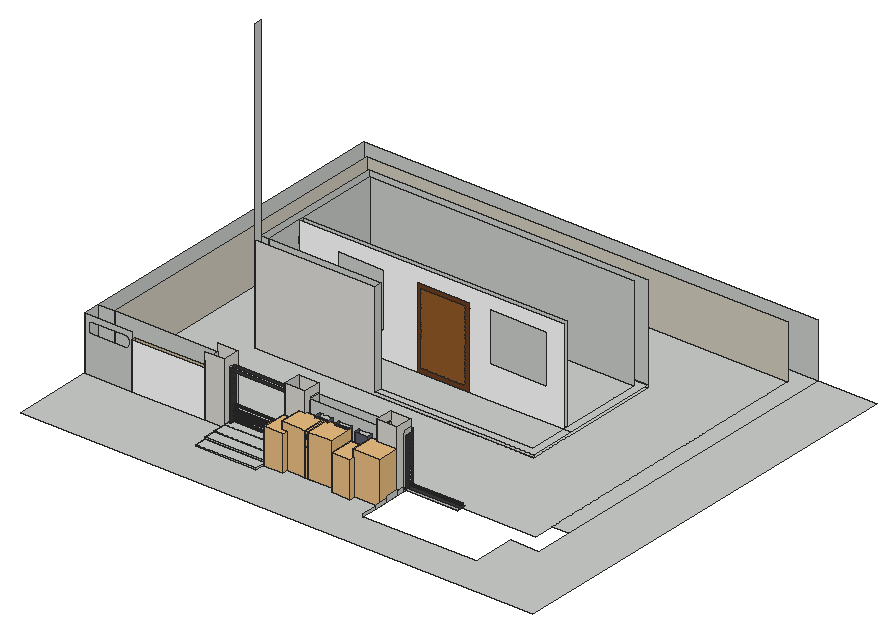
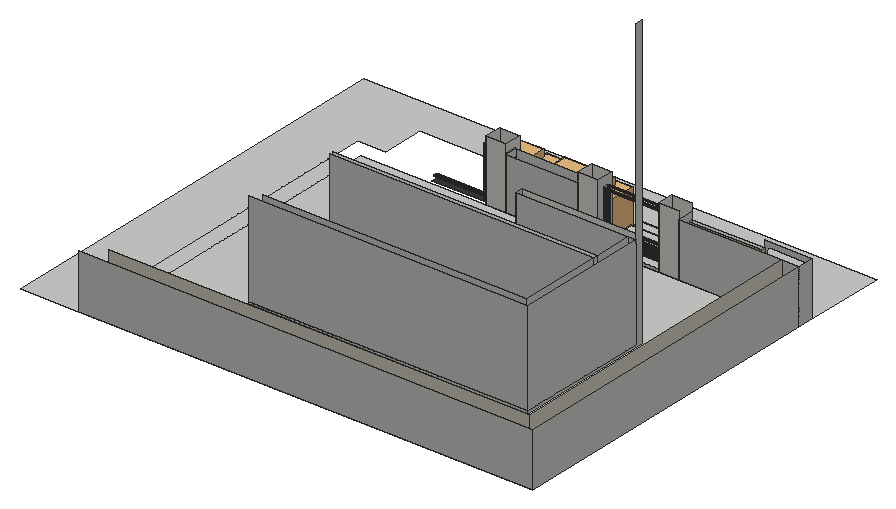
# SketchUp Ruby script. Lengths in inches.
U = 1.inch
M = Sketchup.active_model
def pt(a) = Geom::Point3d.new(a.map { |v| v * U })
def face(e, loops, mat)
  f = e.add_face(loops[0].map { |a| pt(a) })
  loops[1..].each { |l| e.add_face(l.map { |a| pt(a) }).erase! }
  f.material = f.back_material = mat if mat
  f
end
# faces: each face lists its corners as indices into pts; further lists are holes
def faces(e, pts, list, mat = nil) = list.each { |f| face(e, (f[0].is_a?(Array) ? f : [f]).map { |l| l.map { |i| pts[i] } }, mat) }
# xy, xz, yz: faces in a plane at the given z, y or x. An outline is a flat list of corners, or four numbers for a rectangle; further outlines are holes
def ring(l) = l.size == 4 ? [[l[0], l[1]], [l[2], l[1]], [l[2], l[3]], [l[0], l[3]]] : l.each_slice(2).to_a
def flat(e, list, mat, &to3) = list.each { |f| face(e, (f[0].is_a?(Array) ? f : [f]).map { |l| ring(l).map { |u, v| to3.(u, v) } }, mat) }
def xy(e, z, list, mat = nil) = flat(e, list, mat) { |x, y| [x, y, z] }
def xz(e, y, list, mat = nil) = flat(e, list, mat) { |x, z| [x, y, z] }
def yz(e, x, list, mat = nil) = flat(e, list, mat) { |y, z| [x, y, z] }
def lines(e, pts, list) = list.each { |a, b| e.add_line(pt(pts[a]), pt(pts[b])) }
# prism: a flat outline (further loops are holes) pulled along v
def prism(e, loops, v, mat = nil)
  f = face(e, loops, mat); d = Geom::Vector3d.new(v.map { |x| x * U })
  f.pushpull(f.normal.samedirection?(d) ? d.length : -d.length)
end
def box(e, o, s, mat = nil) = prism(e, [[o, [o[0] + s[0], o[1], o[2]], [o[0] + s[0], o[1] + s[1], o[2]], [o[0], o[1] + s[1], o[2]]]], [0, 0, s[2]], mat)
def at(x, y, z, deg = 0) = Geom::Transformation.translation(pt([x, y, z])) * Geom::Transformation.rotation(ORIGIN, Z_AXIS, deg.degrees)
def axes(o, x, y, z) = Geom::Transformation.new([*x, 0, *y, 0, *z, 0, *pt(o).to_a, 1])
def part(name) = M.definitions.add(name)
# library, detail: a bought-in or finely detailed component or shape, given as its bounding box
def library(name, o, s) = part(name).tap { |d| box(d.entities, o, s) }
def detail(e, o, s) = box(e.add_group.entities, o, s)
def put(e, d, t, mat = nil) = e.add_instance(d, t).tap { |i| i.material = mat if mat }
def group(e, t, mat = nil) = e.add_group.tap { |g| g.transformation = t; g.material = mat if mat }.entities
root = M.entities
M.materials.add("[Basic Tile]").color = [203, 206, 202]
M.materials.add("[Color M00]").color = [255, 255, 255]
M.materials.add("[Color M07]").color = [58, 58, 58]
M.materials.add("[Formica Graystone]").color = [209, 204, 189]
M.materials.add("[Formica Laminate Dark]").color = [89, 94, 107]
M.materials.add("[Quartz Light Brown]").color = [199, 184, 152]
M.materials.add("[Terrazzo Tile Accent]").color = [224, 221, 217]
M.materials.add("[Terrazzo Tile Light]").color = [219, 217, 210]
M.materials.add("[Wood Floor Parquet]").color = [145, 89, 39]
M.materials.add("[Wood Veneer 01]").color = [107, 62, 33]
c1 = library("chau cay",[-24.34,-109.24,0],[56.46,62.58,79.69])
c2 = library("Flora+17",[-57.52,158.6,-38.64],[66.99,62.88,77.28])
xy(root,0,[[0,0,0,289.93,504.35,289.93,504.35,159.78,722.52,159.78,722.52,289.93,1126.47,289.93,1126.47,137.11,1535.88,137.11,1535.88,289.93,1639.03,289.93,1639.03,1547.14,1848.64,1547.14,1848.64,0],[504.35,159.78,722.52,201.53],[504.35,201.53,722.52,243.28],[504.35,243.28,722.52,289.93],[0,289.93,0,350.55,431.58,350.55,431.58,303.99,171.04,303.99,171.04,289.93],
  [171.04,289.93,431.58,303.99],[431.58,289.93,504.35,350.55],[504.35,289.93,722.52,350.55],[722.52,289.93,795.29,350.55],[795.29,289.93,1053.71,309.57],
  [1053.71,289.93,1126.47,350.55],[795.29,309.57,1053.71,350.55],[0,350.55,0,1547.14,1639.03,1547.14,1639.03,424.2,1578.42,424.2,1578.42,1486.52,60.61,1486.52,60.61,350.55],[[60.61,350.55,1578.42,1486.52],[282.77,703.09,1290.28,1215.04]],[282.77,703.09,1290.28,1215.04]],"[Basic Tile]")
xy(root,4.4375,[[504.35,159.78,722.52,201.53]],"[Basic Tile]")
xy(root,6.25,[[504.35,307.1,513.6,328.82],[716.4,307.1,722.52,328.82]],"[Basic Tile]")
xy(root,8.3125,[[1126.47,320.24,1134.85,350.55]],"[Basic Tile]")
xy(root,8.3125,[[1134.85,320.24,1322.28,350.55]],"[Color M07]")
xy(root,9,[[716.67,703.09,1290.28,703.09,1290.28,868.79,1262.85,868.79,1262.85,730.52,716.67,730.52],[282.77,730.52,282.77,1215.04,1290.28,1215.04,1290.28,868.79,1262.85,868.79,1262.85,1187.61,310.19,1187.61,310.19,730.52],[310.19,730.52,1262.85,868.79],[310.19,868.79,1262.85,886.125],[310.19,886.125,1262.85,1187.61]],"[Basic Tile]")
xy(root,10,[[504.35,201.53,722.52,243.28]],"[Basic Tile]")
xy(root,12.0625,[[504.35,243.28,722.52,289.93],[504.35,289.93,722.52,289.93,722.52,307.1,716.4,307.1,716.4,328.82,722.52,328.82,722.52,350.55,504.35,350.55,504.35,328.82,513.6,328.82,513.6,307.1,504.35,307.1]],"[Basic Tile]")
xy(root,32.19,[[832.8125,288.14,879.5,309.57],[902.5,288.14,949.1875,309.57],[974.4375,288.14,1021.125,309.57]],"[Formica Laminate Dark]")
xz(root,159.78,[[504.35,0,722.52,4.4375]],"[Basic Tile]")
xz(root,201.53,[[504.35,0,722.52,4.4375],[504.35,4.4375,722.52,10]],"[Basic Tile]")
xz(root,243.28,[[504.35,0,722.52,10],[504.35,10,722.52,12.0625]],"[Basic Tile]")
xz(root,288.14,[[832.8125,32.19,879.5,155.26],[902.5,32.19,949.1875,155.26],[974.4375,32.19,1021.125,155.26]],"[Formica Laminate Dark]")
xz(root,289.93,[[[0,0,171.04,194.8125],[23.08,135.12,21.82,135.21,20.58,135.45,19.38,135.86,18.25,136.42,17.2,137.12,16.25,137.95,15.42,138.9,14.72,139.95,14.16,141.08,13.76,142.27,13.51,143.51,13.43,144.77,13.43,162.96,13.54,164.66,13.87,166.32,14.42,167.93,15.17,169.45,16.11,170.86,17.23,172.14,18.5,173.25,19.91,174.2,21.4375,174.95,23.04,175.49,24.71,175.82,26.4,175.94,148.48,175.94,150.17,175.82,151.83,175.49,153.4375,174.95,154.96,174.2,156.36,173.26,157.64,172.14,158.75,170.87,159.69,169.46,160.44,167.94,160.99,166.34,161.32,164.68,161.43,162.99,161.43,147.17,161.32,145.6,161.02,144.05,160.51,142.56,159.8125,141.15,158.9375,139.84,157.9,138.65,156.71,137.61,155.4,136.74,153.99,136.04,152.5,135.53,150.95,135.23,149.38,135.12]],[504.35,0,722.52,12.0625]],"[Basic Tile]")
xz(root,289.93,[[171.04,0,431.58,168.17]],"[Color M00]")
xz(root,289.93,[[431.58,0,504.35,222.4375],[722.52,0,795.29,222.4375],[1053.71,0,1126.47,222.4375]],"[Terrazzo Tile Light]")
xz(root,303.99,[[171.04,0,431.58,168.17]],"[Quartz Light Brown]")
xz(root,307.1,[[504.35,6.25,513.6,12.0625],[716.4,6.25,722.52,12.0625]],"[Basic Tile]")
xz(root,307.1,[[504.35,12.0625,513.6,12.0625,513.6,180.91,716.4,180.91,716.4,12.0625,722.52,12.0625,722.52,190.375,504.35,190.375]],"[Color M07]")
xz(root,309.57,[[832.8125,32.19,879.5,155.26],[902.5,32.19,949.1875,155.26],[974.4375,32.19,1021.125,155.26]])
xz(root,309.57,[[[795.29,0,1053.71,186.9375],[832.8125,32.19,879.5,155.26],[902.5,32.19,949.1875,155.26],[974.4375,32.19,1021.125,155.26]]],"[Basic Tile]")
xz(root,320.24,[[1134.85,8.3125,1322.28,15.5]],"[Basic Tile]")
xz(root,320.24,[[1126.47,8.3125,1134.85,15.5]],"[Color M07]")
xz(root,328.82,[[504.35,6.25,513.6,12.0625],[716.4,6.25,722.52,12.0625]],"[Basic Tile]")
xz(root,328.82,[[504.35,12.0625,513.6,190.375],[716.4,12.0625,716.4,180.91,513.6,180.91,513.6,190.375,722.52,190.375,722.52,12.0625]],"[Color M07]")
xz(root,350.55,[[0,0,60.61,194.8125],[60.61,0,431.58,194.8125],[504.35,0,722.52,12.0625],[795.29,0,1053.71,186.9375]],"[Basic Tile]")
xz(root,350.55,[[1126.47,8.3125,1134.85,195.17]],"[Color M07]")
xz(root,350.55,[[431.58,0,504.35,222.4375],[722.52,0,795.29,222.4375],[1053.71,0,1126.47,222.4375]],"[Terrazzo Tile Light]")
xz(root,703.09,[[282.77,0,1290.28,0,1290.28,9,716.67,9,716.67,349.625,282.77,349.625]],"[Terrazzo Tile Accent]")
xz(root,730.52,[[282.77,9,310.19,349.625],[310.19,9,716.67,349.625]],"[Basic Tile]")
xz(root,868.79,[[[310.19,9,733.48,9,733.48,299.625,925.73,299.625,925.73,9,1262.85,9,1262.85,349.625,310.19,349.625],[996.55,125.8125,1202.24,302.9375],[448.22,100.38,615.78,297.32]]],"[Color M00]")
xz(root,868.79,[[749.83,25.35,909.375,283.28]],"[Wood Floor Parquet]")
xz(root,868.79,[[[733.48,9,925.73,299.625],[749.83,25.35,909.375,283.28]]],"[Wood Veneer 01]")
xz(root,886.125,[[310.19,9,1262.85,349.625]],"[Basic Tile]")
xz(root,1187.61,[[310.19,9,1262.85,349.625]],"[Basic Tile]")
xz(root,1215.04,[[282.77,0,1290.28,9],[282.77,9,1290.28,349.625]],"[Basic Tile]")
xz(root,1486.52,[[60.61,0,1578.42,194.8125]],"[Formica Graystone]")
xz(root,1547.14,[[0,0,1639.03,194.8125]],"[Basic Tile]")
yz(root,0,[[289.93,0,350.55,194.8125],[350.55,0,1547.14,194.8125]],"[Basic Tile]")
yz(root,60.61,[[350.55,0,1486.52,194.8125]],"[Formica Graystone]")
yz(root,171.04,[[289.93,0,303.99,168.17]],"[Quartz Light Brown]")
yz(root,282.77,[[703.09,0,703.09,1047.125,730.52,1047.125,730.52,9,1215.04,9,1215.04,0],[730.52,9,1215.04,349.625]],"[Basic Tile]")
yz(root,310.19,[[730.52,9,868.79,349.625],[868.79,9,886.125,349.625],[886.125,9,1187.61,349.625]],"[Basic Tile]")
yz(root,431.58,[[289.93,0,303.99,168.17],[303.99,0,350.55,0,350.55,194.8125,289.93,194.8125,289.93,168.17,303.99,168.17]],"[Basic Tile]")
yz(root,504.35,[[159.78,0,201.53,4.4375],[201.53,0,243.28,10],[243.28,0,289.93,12.0625],[289.93,0,350.55,0,350.55,12.0625,328.82,12.0625,328.82,6.25,307.1,6.25,307.1,12.0625,289.93,12.0625],[307.1,6.25,328.82,190.375]],"[Basic Tile]")
yz(root,504.35,[[289.93,12.0625,307.1,12.0625,307.1,190.375,328.82,190.375,328.82,12.0625,350.55,12.0625,350.55,222.4375,289.93,222.4375]],"[Terrazzo Tile Light]")
yz(root,513.6,[[307.1,6.25,328.82,12.0625]],"[Basic Tile]")
yz(root,513.6,[[[307.1,12.0625,328.82,180.91],[319.3,161.86,318.3,162,317.37,162.38,316.56,163,315.95,163.8,315.5625,164.74,315.43,165.74,315.5625,166.74,315.95,167.68,316.56,168.48,317.37,169.09,318.3,169.48,319.3,169.61,320.31,169.48,321.24,169.09,322.04,168.48,322.66,167.68,323.05,166.74,323.18,165.74,323.05,164.74,322.66,163.8,322.04,163,321.24,162.38,320.31,162],[319.3,144.8,318.3,144.93,317.37,145.32,316.56,145.9375,315.95,146.74,315.5625,147.67,315.43,148.68,315.5625,149.68,315.95,150.61,316.56,151.42,317.37,152.03,318.3,152.42,319.3,152.55,320.31,152.42,321.24,152.03,322.04,151.42,322.66,150.61,323.05,149.68,323.18,148.68,323.05,147.67,322.66,146.74,322.04,145.9375,321.24,145.32,320.31,144.93],[319.3,129.24,318.3,129.37,317.37,129.76,316.56,130.375,315.95,131.18,315.5625,132.11,315.43,133.11,315.5625,134.12,315.95,135.05,316.56,135.85,317.37,136.47,318.3,136.86,319.3,136.99,320.31,136.86,321.24,136.47,322.04,135.85,322.66,135.05,323.05,134.12,323.18,133.11,323.05,132.11,322.66,131.18,322.04,130.375,321.24,129.76,320.31,129.37],[319.3,113.8,318.3,113.93,317.37,114.32,316.56,114.9375,315.95,115.74,315.5625,116.67,315.43,117.68,315.5625,118.68,315.95,119.61,316.56,120.42,317.37,121.03,318.3,121.42,319.3,121.55,320.31,121.42,321.24,121.03,322.04,120.42,322.66,119.61,323.05,118.68,323.18,117.68,323.05,116.67,322.66,115.74,322.04,114.9375,321.24,114.32,320.31,113.93],[319.3,99.55,318.3,99.68,317.37,100.07,316.56,100.6875,315.95,101.49,315.5625,102.42,315.43,103.43,315.5625,104.43,315.95,105.36,316.56,106.17,317.37,106.78,318.3,107.17,319.3,107.3,320.31,107.17,321.24,106.78,322.04,106.17,322.66,105.36,323.05,104.43,323.18,103.43,323.05,102.42,322.66,101.49,322.04,100.6875,321.24,100.07,320.31,99.68],[319.3,81.86,318.3,82,317.37,82.38,316.56,83,315.95,83.8,315.5625,84.74,315.43,85.74,315.5625,86.74,315.95,87.68,316.56,88.48,317.37,89.09,318.3,89.48,319.3,89.61,320.31,89.48,321.24,89.09,322.04,88.48,322.66,87.68,323.05,86.74,323.18,85.74,323.05,84.74,322.66,83.8,322.04,83,321.24,82.38,320.31,82],[319.3,64.86,318.3,65,317.37,65.38,316.56,66,315.95,66.8,315.5625,67.74,315.43,68.74,315.5625,69.74,315.95,70.68,316.56,71.48,317.37,72.09,318.3,72.48,319.3,72.61,320.31,72.48,321.24,72.09,322.04,71.48,322.66,70.68,323.05,69.74,323.18,68.74,323.05,67.74,322.66,66.8,322.04,66,321.24,65.38,320.31,65],[319.3,13.93,318.3,14.06,317.37,14.45,316.56,15.0625,315.95,15.86,315.5625,16.8,315.43,17.8,315.5625,18.8,315.95,19.74,316.56,20.54,317.37,21.16,318.3,21.54,319.3,21.68,320.31,21.54,321.24,21.16,322.04,20.54,322.66,19.74,323.05,18.8,323.18,17.8,323.05,16.8,322.66,15.86,322.04,15.0625,321.24,14.45,320.31,14.06],[319.3,30.55,318.3,30.68,317.37,31.07,316.56,31.6875,315.95,32.49,315.5625,33.42,315.43,34.43,315.5625,35.43,315.95,36.36,316.56,37.17,317.37,37.78,318.3,38.17,319.3,38.3,320.31,38.17,321.24,37.78,322.04,37.17,322.66,36.36,323.05,35.43,323.18,34.43,323.05,33.42,322.66,32.49,322.04,31.6875,321.24,31.07,320.31,30.68],[319.3,46.86,318.3,47,317.37,47.38,316.56,48,315.95,48.8,315.5625,49.74,315.43,50.74,315.5625,51.74,315.95,52.68,316.56,53.48,317.37,54.09,318.3,54.48,319.3,54.61,320.31,54.48,321.24,54.09,322.04,53.48,322.66,52.68,323.05,51.74,323.18,50.74,323.05,49.74,322.66,48.8,322.04,48,321.24,47.38,320.31,47]]],"[Color M07]")
yz(root,716.4,[[319.3,13.93,320.31,14.06,321.24,14.45,322.04,15.0625,322.66,15.86,323.05,16.8,323.18,17.8,323.05,18.8,322.66,19.74,322.04,20.54,321.24,21.16,320.31,21.54,319.3,21.68,318.3,21.54,317.37,21.16,316.56,20.54,315.95,19.74,315.5625,18.8,315.43,17.8,315.5625,16.8,315.95,15.86,316.56,15.0625,317.37,14.45,318.3,14.06],[319.3,30.55,320.31,30.68,321.24,31.07,322.04,31.6875,322.66,32.49,323.05,33.42,323.18,34.43,323.05,35.43,322.66,36.36,322.04,37.17,321.24,37.78,320.31,38.17,319.3,38.3,318.3,38.17,317.37,37.78,316.56,37.17,315.95,36.36,315.5625,35.43,315.43,34.43,315.5625,33.42,315.95,32.49,316.56,31.6875,317.37,31.07,318.3,30.68],[319.3,46.86,320.31,47,321.24,47.38,322.04,48,322.66,48.8,323.05,49.74,323.18,50.74,323.05,51.74,322.66,52.68,322.04,53.48,321.24,54.09,320.31,54.48,319.3,54.61,318.3,54.48,317.37,54.09,316.56,53.48,315.95,52.68,315.5625,51.74,315.43,50.74,315.5625,49.74,315.95,48.8,316.56,48,317.37,47.38,318.3,47],[319.3,64.86,320.31,65,321.24,65.38,322.04,66,322.66,66.8,323.05,67.74,323.18,68.74,323.05,69.74,322.66,70.68,322.04,71.48,321.24,72.09,320.31,72.48,319.3,72.61,318.3,72.48,317.37,72.09,316.56,71.48,315.95,70.68,315.5625,69.74,315.43,68.74,315.5625,67.74,315.95,66.8,316.56,66,317.37,65.38,318.3,65]])
yz(root,716.4,[[307.1,6.25,328.82,12.0625]],"[Basic Tile]")
yz(root,716.4,[[[307.1,12.0625,328.82,180.91],[319.3,161.86,320.31,162,321.24,162.38,322.04,163,322.66,163.8,323.05,164.74,323.18,165.74,323.05,166.74,322.66,167.68,322.04,168.48,321.24,169.09,320.31,169.48,319.3,169.61,318.3,169.48,317.37,169.09,316.56,168.48,315.95,167.68,315.5625,166.74,315.43,165.74,315.5625,164.74,315.95,163.8,316.56,163,317.37,162.38,318.3,162],[319.3,13.93,320.31,14.06,321.24,14.45,322.04,15.0625,322.66,15.86,323.05,16.8,323.18,17.8,323.05,18.8,322.66,19.74,322.04,20.54,321.24,21.16,320.31,21.54,319.3,21.68,318.3,21.54,317.37,21.16,316.56,20.54,315.95,19.74,315.5625,18.8,315.43,17.8,315.5625,16.8,315.95,15.86,316.56,15.0625,317.37,14.45,318.3,14.06],[319.3,144.8,320.31,144.93,321.24,145.32,322.04,145.9375,322.66,146.74,323.05,147.67,323.18,148.68,323.05,149.68,322.66,150.61,322.04,151.42,321.24,152.03,320.31,152.42,319.3,152.55,318.3,152.42,317.37,152.03,316.56,151.42,315.95,150.61,315.5625,149.68,315.43,148.68,315.5625,147.67,315.95,146.74,316.56,145.9375,317.37,145.32,318.3,144.93],[319.3,30.55,320.31,30.68,321.24,31.07,322.04,31.6875,322.66,32.49,323.05,33.42,323.18,34.43,323.05,35.43,322.66,36.36,322.04,37.17,321.24,37.78,320.31,38.17,319.3,38.3,318.3,38.17,317.37,37.78,316.56,37.17,315.95,36.36,315.5625,35.43,315.43,34.43,315.5625,33.42,315.95,32.49,316.56,31.6875,317.37,31.07,318.3,30.68],[319.3,129.24,320.31,129.37,321.24,129.76,322.04,130.375,322.66,131.18,323.05,132.11,323.18,133.11,323.05,134.12,322.66,135.05,322.04,135.85,321.24,136.47,320.31,136.86,319.3,136.99,318.3,136.86,317.37,136.47,316.56,135.85,315.95,135.05,315.5625,134.12,315.43,133.11,315.5625,132.11,315.95,131.18,316.56,130.375,317.37,129.76,318.3,129.37],[319.3,46.86,320.31,47,321.24,47.38,322.04,48,322.66,48.8,323.05,49.74,323.18,50.74,323.05,51.74,322.66,52.68,322.04,53.48,321.24,54.09,320.31,54.48,319.3,54.61,318.3,54.48,317.37,54.09,316.56,53.48,315.95,52.68,315.5625,51.74,315.43,50.74,315.5625,49.74,315.95,48.8,316.56,48,317.37,47.38,318.3,47],[319.3,113.8,320.31,113.93,321.24,114.32,322.04,114.9375,322.66,115.74,323.05,116.67,323.18,117.68,323.05,118.68,322.66,119.61,322.04,120.42,321.24,121.03,320.31,121.42,319.3,121.55,318.3,121.42,317.37,121.03,316.56,120.42,315.95,119.61,315.5625,118.68,315.43,117.68,315.5625,116.67,315.95,115.74,316.56,114.9375,317.37,114.32,318.3,113.93],[319.3,64.86,320.31,65,321.24,65.38,322.04,66,322.66,66.8,323.05,67.74,323.18,68.74,323.05,69.74,322.66,70.68,322.04,71.48,321.24,72.09,320.31,72.48,319.3,72.61,318.3,72.48,317.37,72.09,316.56,71.48,315.95,70.68,315.5625,69.74,315.43,68.74,315.5625,67.74,315.95,66.8,316.56,66,317.37,65.38,318.3,65],[319.3,99.55,320.31,99.68,321.24,100.07,322.04,100.6875,322.66,101.49,323.05,102.42,323.18,103.43,323.05,104.43,322.66,105.36,322.04,106.17,321.24,106.78,320.31,107.17,319.3,107.3,318.3,107.17,317.37,106.78,316.56,106.17,315.95,105.36,315.5625,104.43,315.43,103.43,315.5625,102.42,315.95,101.49,316.56,100.6875,317.37,100.07,318.3,99.68],[319.3,81.86,320.31,82,321.24,82.38,322.04,83,322.66,83.8,323.05,84.74,323.18,85.74,323.05,86.74,322.66,87.68,322.04,88.48,321.24,89.09,320.31,89.48,319.3,89.61,318.3,89.48,317.37,89.09,316.56,88.48,315.95,87.68,315.5625,86.74,315.43,85.74,315.5625,84.74,315.95,83.8,316.56,83,317.37,82.38,318.3,82]]],"[Color M07]")
yz(root,716.67,[[703.09,9,730.52,349.625]],"[Basic Tile]")
yz(root,717.58,[[319.3,46.86,320.31,47,321.24,47.38,322.04,48,322.66,48.8,323.05,49.74,323.18,50.74,323.05,51.74,322.66,52.68,322.04,53.48,321.24,54.09,320.31,54.48,319.3,54.61,318.3,54.48,317.37,54.09,316.56,53.48,315.95,52.68,315.5625,51.74,315.43,50.74,315.5625,49.74,315.95,48.8,316.56,48,317.37,47.38,318.3,47]])
yz(root,722.52,[[159.78,0,201.53,4.4375],[201.53,0,243.28,10],[243.28,0,289.93,12.0625],[289.93,0,289.93,12.0625,307.1,12.0625,307.1,6.25,328.82,6.25,328.82,12.0625,350.55,12.0625,350.55,0],[307.1,6.25,328.82,190.375],
  [289.93,12.0625,289.93,222.4375,350.55,222.4375,350.55,12.0625,328.82,12.0625,328.82,190.375,307.1,190.375,307.1,12.0625]],"[Basic Tile]")
yz(root,795.29,[[309.57,0,350.55,186.9375]],"[Basic Tile]")
yz(root,795.29,[[289.93,0,309.57,0,309.57,193.9375,350.55,193.9375,350.55,222.4375,289.93,222.4375]],"[Terrazzo Tile Light]")
yz(root,832.8125,[[288.14,32.19,309.57,155.26]],"[Formica Laminate Dark]")
yz(root,879.5,[[288.14,32.19,309.57,155.26]],"[Formica Laminate Dark]")
yz(root,902.5,[[288.14,32.19,309.57,155.26]],"[Formica Laminate Dark]")
yz(root,949.1875,[[288.14,32.19,309.57,155.26]],"[Formica Laminate Dark]")
yz(root,974.4375,[[288.14,32.19,309.57,155.26]],"[Formica Laminate Dark]")
yz(root,1021.125,[[288.14,32.19,309.57,155.26]],"[Formica Laminate Dark]")
yz(root,1053.71,[[309.57,0,350.55,186.9375]],"[Basic Tile]")
yz(root,1053.71,[[289.93,0,289.93,222.4375,350.55,222.4375,350.55,193.9375,309.57,193.9375,309.57,0]],"[Terrazzo Tile Light]")
yz(root,1126.47,[[137.11,0,187.89,8.4375],[187.89,0,238.67,11.8125],[238.67,0,289.93,17.75],[289.93,0,320.24,15.5],[320.24,0,350.55,8.3125],
  [320.24,8.3125,350.55,195.17]],"[Basic Tile]")
yz(root,1126.47,[[289.93,15.5,320.24,15.5,320.24,195.17,350.55,195.17,350.55,222.4375,289.93,222.4375]],"[Terrazzo Tile Light]")
yz(root,1134.85,[[337.34,16.89,336.35,17.02,335.43,17.4,334.65,18.01,334.04,18.8,333.66,19.72,333.53,20.71,333.66,21.69,334.04,22.61,334.65,23.4,335.43,24.01,336.35,24.39,337.34,24.52,338.33,24.39,339.25,24.01,340.04,23.4,340.64,22.61,341.02,21.69,341.15,20.71,341.02,19.72,340.64,18.8,340.04,18.01,339.25,17.4,338.33,17.02],[337.34,31.39,336.35,31.52,335.43,31.9,334.65,32.51,334.04,33.3,333.66,34.22,333.53,35.21,333.66,36.19,334.04,37.11,334.65,37.9,335.43,38.51,336.35,38.89,337.34,39.02,338.33,38.89,339.25,38.51,340.04,37.9,340.64,37.11,341.02,36.19,341.15,35.21,341.02,34.22,340.64,33.3,340.04,32.51,339.25,31.9,338.33,31.52],[337.34,47.21,336.35,47.34,335.43,47.72,334.65,48.32,334.04,49.11,333.66,50.03,333.53,51.02,333.66,52,334.04,52.92,334.65,53.71,335.43,54.32,336.35,54.7,337.34,54.83,338.33,54.7,339.25,54.32,340.04,53.71,340.64,52.92,341.02,52,341.15,51.02,341.02,50.03,340.64,49.11,340.04,48.32,339.25,47.72,338.33,47.34],[337.34,61.64,336.35,61.77,335.43,62.15,334.65,62.76,334.04,63.55,333.66,64.47,333.53,65.46,333.66,66.44,334.04,67.36,334.65,68.15,335.43,68.76,336.35,69.14,337.34,69.27,338.33,69.14,339.25,68.76,340.04,68.15,340.64,67.36,341.02,66.44,341.15,65.46,341.02,64.47,340.64,63.55,340.04,62.76,339.25,62.15,338.33,61.77]])
yz(root,1134.85,[[[320.24,8.3125,350.55,184.74],[337.34,174.52,336.35,174.65,335.43,175.03,334.65,175.63,334.04,176.42,333.66,177.34,333.53,178.33,333.66,179.32,334.04,180.24,334.65,181.03,335.43,181.63,336.35,182.01,337.34,182.14,338.33,182.01,339.25,181.63,340.04,181.03,340.64,180.24,341.02,179.32,341.15,178.33,341.02,177.34,340.64,176.42,340.04,175.63,339.25,175.03,338.33,174.65],[337.34,161.02,336.35,161.15,335.43,161.53,334.65,162.13,334.04,162.92,333.66,163.84,333.53,164.83,333.66,165.82,334.04,166.74,334.65,167.53,335.43,168.13,336.35,168.51,337.34,168.64,338.33,168.51,339.25,168.13,340.04,167.53,340.64,166.74,341.02,165.82,341.15,164.83,341.02,163.84,340.64,162.92,340.04,162.13,339.25,161.53,338.33,161.15],[337.34,147.52,336.35,147.65,335.43,148.03,334.65,148.63,334.04,149.42,333.66,150.34,333.53,151.33,333.66,152.32,334.04,153.24,334.65,154.03,335.43,154.63,336.35,155.01,337.34,155.14,338.33,155.01,339.25,154.63,340.04,154.03,340.64,153.24,341.02,152.32,341.15,151.33,341.02,150.34,340.64,149.42,340.04,148.63,339.25,148.03,338.33,147.65],[337.34,134.02,336.35,134.15,335.43,134.53,334.65,135.13,334.04,135.92,333.66,136.84,333.53,137.83,333.66,138.82,334.04,139.74,334.65,140.53,335.43,141.13,336.35,141.51,337.34,141.64,338.33,141.51,339.25,141.13,340.04,140.53,340.64,139.74,341.02,138.82,341.15,137.83,341.02,136.84,340.64,135.92,340.04,135.13,339.25,134.53,338.33,134.15],[337.34,117.89,336.35,118.02,335.43,118.4,334.65,119.01,334.04,119.8,333.66,120.72,333.53,121.71,333.66,122.69,334.04,123.61,334.65,124.4,335.43,125.01,336.35,125.39,337.34,125.52,338.33,125.39,339.25,125.01,340.04,124.4,340.64,123.61,341.02,122.69,341.15,121.71,341.02,120.72,340.64,119.8,340.04,119.01,339.25,118.4,338.33,118.02],[337.34,103.39,336.35,103.52,335.43,103.9,334.65,104.51,334.04,105.3,333.66,106.22,333.53,107.21,333.66,108.19,334.04,109.11,334.65,109.9,335.43,110.51,336.35,110.89,337.34,111.02,338.33,110.89,339.25,110.51,340.04,109.9,340.64,109.11,341.02,108.19,341.15,107.21,341.02,106.22,340.64,105.3,340.04,104.51,339.25,103.9,338.33,103.52],[337.34,90.83,336.35,90.96,335.43,91.34,334.65,91.95,334.04,92.74,333.66,93.66,333.53,94.64,333.66,95.63,334.04,96.55,334.65,97.34,335.43,97.94,336.35,98.33,337.34,98.46,338.33,98.33,339.25,97.94,340.04,97.34,340.64,96.55,341.02,95.63,341.15,94.64,341.02,93.66,340.64,92.74,340.04,91.95,339.25,91.34,338.33,90.96],[337.34,76.33,336.35,76.46,335.43,76.84,334.65,77.45,334.04,78.24,333.66,79.16,333.53,80.14,333.66,81.13,334.04,82.05,334.65,82.84,335.43,83.44,336.35,83.83,337.34,83.96,338.33,83.83,339.25,83.44,340.04,82.84,340.64,82.05,341.02,81.13,341.15,80.14,341.02,79.16,340.64,78.24,340.04,77.45,339.25,76.84,338.33,76.46],[337.34,61.64,336.35,61.77,335.43,62.15,334.65,62.76,334.04,63.55,333.66,64.47,333.53,65.46,333.66,66.44,334.04,67.36,334.65,68.15,335.43,68.76,336.35,69.14,337.34,69.27,338.33,69.14,339.25,68.76,340.04,68.15,340.64,67.36,341.02,66.44,341.15,65.46,341.02,64.47,340.64,63.55,340.04,62.76,339.25,62.15,338.33,61.77],[337.34,47.21,336.35,47.34,335.43,47.72,334.65,48.32,334.04,49.11,333.66,50.03,333.53,51.02,333.66,52,334.04,52.92,334.65,53.71,335.43,54.32,336.35,54.7,337.34,54.83,338.33,54.7,339.25,54.32,340.04,53.71,340.64,52.92,341.02,52,341.15,51.02,341.02,50.03,340.64,49.11,340.04,48.32,339.25,47.72,338.33,47.34],[337.34,31.39,336.35,31.52,335.43,31.9,334.65,32.51,334.04,33.3,333.66,34.22,333.53,35.21,333.66,36.19,334.04,37.11,334.65,37.9,335.43,38.51,336.35,38.89,337.34,39.02,338.33,38.89,339.25,38.51,340.04,37.9,340.64,37.11,341.02,36.19,341.15,35.21,341.02,34.22,340.64,33.3,340.04,32.51,339.25,31.9,338.33,31.52],[337.34,16.89,336.35,17.02,335.43,17.4,334.65,18.01,334.04,18.8,333.66,19.72,333.53,20.71,333.66,21.69,334.04,22.61,334.65,23.4,335.43,24.01,336.35,24.39,337.34,24.52,338.33,24.39,339.25,24.01,340.04,23.4,340.64,22.61,341.02,21.69,341.15,20.71,341.02,19.72,340.64,18.8,340.04,18.01,339.25,17.4,338.33,17.02]]],"[Color M07]")
p = [[716.4,319.3,13.93],[716.4,318.3,14.06],[513.6,318.3,14.06],[513.6,319.3,13.93],[716.4,320.31,14.06],[513.6,320.31,14.06],
  [716.4,317.37,14.45],[513.6,317.37,14.45],[716.4,321.24,14.45],[513.6,321.24,14.45],[716.4,316.56,15.0625],[513.6,316.56,15.0625],
  [716.4,322.04,15.0625],[513.6,322.04,15.0625],[716.4,315.95,15.86],[513.6,315.95,15.86],[716.4,322.66,15.86],[513.6,322.66,15.86],
  [716.4,315.5625,16.8],[513.6,315.5625,16.8],[716.4,323.05,16.8],[513.6,323.05,16.8],[716.4,315.43,17.8],[513.6,315.43,17.8],
  [716.4,323.18,17.8],[513.6,323.18,17.8],[1134.85,336.35,17.02],[1134.85,337.34,16.89],[1322.28,337.34,16.89],[1322.28,336.35,17.02],
  [1134.85,338.33,17.02],[1322.28,338.33,17.02],[1134.85,335.43,17.4],[1322.28,335.43,17.4],[1134.85,339.25,17.4],[1322.28,339.25,17.4],
  [1134.85,334.65,18.01],[1322.28,334.65,18.01],[1134.85,340.04,18.01],[1322.28,340.04,18.01],[716.4,315.5625,18.8],[513.6,315.5625,18.8],
  [716.4,323.05,18.8],[513.6,323.05,18.8],[1134.85,334.04,18.8],[1322.28,334.04,18.8],[1134.85,340.64,18.8],[1322.28,340.64,18.8],
  [716.4,315.95,19.74],[513.6,315.95,19.74],[716.4,322.66,19.74],[513.6,322.66,19.74],[1134.85,333.66,19.72],[1322.28,333.66,19.72],
  [1134.85,341.02,19.72],[1322.28,341.02,19.72],[716.4,316.56,20.54],[513.6,316.56,20.54],[716.4,322.04,20.54],[513.6,322.04,20.54],
  [1134.85,333.53,20.71],[1322.28,333.53,20.71],[1134.85,341.15,20.71],[1322.28,341.15,20.71],[716.4,317.37,21.16],[513.6,317.37,21.16],
  [716.4,321.24,21.16],[513.6,321.24,21.16],[1134.85,333.66,21.69],[1322.28,333.66,21.69],[1134.85,341.02,21.69],[1322.28,341.02,21.69],
  [716.4,318.3,21.54],[513.6,318.3,21.54],[716.4,320.31,21.54],[513.6,320.31,21.54],[716.4,319.3,21.68],[513.6,319.3,21.68],
  [1134.85,334.04,22.61],[1322.28,334.04,22.61],[1134.85,340.64,22.61],[1322.28,340.64,22.61],[1134.85,334.65,23.4],[1322.28,334.65,23.4],
  [1134.85,340.04,23.4],[1322.28,340.04,23.4],[716.4,319.3,30.55],[716.4,318.3,30.68],[513.6,318.3,30.68],[513.6,319.3,30.55],
  [716.4,320.31,30.68],[513.6,320.31,30.68],[716.4,317.37,31.07],[513.6,317.37,31.07],[716.4,321.24,31.07],[513.6,321.24,31.07],
  [716.4,316.56,31.6875],[513.6,316.56,31.6875],[716.4,322.04,31.6875],[513.6,322.04,31.6875],[716.4,315.95,32.49],[513.6,315.95,32.49],
  [716.4,322.66,32.49],[513.6,322.66,32.49],[716.4,315.5625,33.42],[513.6,315.5625,33.42],[716.4,323.05,33.42],[513.6,323.05,33.42],
  [716.4,315.43,34.43],[513.6,315.43,34.43],[716.4,323.18,34.43],[513.6,323.18,34.43],[716.4,315.5625,35.43],[513.6,315.5625,35.43],
  [716.4,323.05,35.43],[513.6,323.05,35.43],[716.4,315.95,36.36],[513.6,315.95,36.36],[716.4,322.66,36.36],[513.6,322.66,36.36],
  [716.4,316.56,37.17],[513.6,316.56,37.17],[716.4,322.04,37.17],[513.6,322.04,37.17],[716.4,317.37,37.78],[513.6,317.37,37.78],
  [716.4,321.24,37.78],[513.6,321.24,37.78],[716.4,318.3,38.17],[513.6,318.3,38.17],[716.4,320.31,38.17],[513.6,320.31,38.17],
  [716.4,319.3,38.3],[513.6,319.3,38.3],[716.4,319.3,46.86],[716.4,318.3,47],[513.6,318.3,47],[513.6,319.3,46.86],
  [717.58,319.3,46.86],[717.58,318.3,47],[716.4,320.31,47],[513.6,320.31,47],[717.58,320.31,47],[716.4,317.37,47.38],
  [513.6,317.37,47.38],[717.58,317.37,47.38],[716.4,321.24,47.38],[513.6,321.24,47.38],[717.58,321.24,47.38],[716.4,316.56,48],
  [513.6,316.56,48],[717.58,316.56,48],[716.4,322.04,48],[513.6,322.04,48],[717.58,322.04,48],[716.4,315.95,48.8],
  [513.6,315.95,48.8],[717.58,315.95,48.8],[716.4,322.66,48.8],[513.6,322.66,48.8],[717.58,322.66,48.8],[716.4,315.5625,49.74],
  [513.6,315.5625,49.74],[717.58,315.5625,49.74],[716.4,323.05,49.74],[513.6,323.05,49.74],[717.58,323.05,49.74],[716.4,315.43,50.74],
  [513.6,315.43,50.74],[717.58,315.43,50.74],[716.4,323.18,50.74],[513.6,323.18,50.74],[717.58,323.18,50.74],[716.4,315.5625,51.74],
  [513.6,315.5625,51.74],[717.58,315.5625,51.74],[716.4,323.05,51.74],[513.6,323.05,51.74],[717.58,323.05,51.74],[716.4,315.95,52.68],
  [513.6,315.95,52.68],[717.58,315.95,52.68],[716.4,322.66,52.68],[513.6,322.66,52.68],[717.58,322.66,52.68],[716.4,316.56,53.48],
  [513.6,316.56,53.48],[717.58,316.56,53.48],[716.4,322.04,53.48],[513.6,322.04,53.48],[717.58,322.04,53.48],[716.4,317.37,54.09],
  [513.6,317.37,54.09],[717.58,317.37,54.09],[716.4,321.24,54.09],[513.6,321.24,54.09],[717.58,321.24,54.09],[716.4,318.3,54.48],
  [513.6,318.3,54.48],[717.58,318.3,54.48],[716.4,320.31,54.48],[513.6,320.31,54.48],[717.58,320.31,54.48],[716.4,319.3,54.61],
  [513.6,319.3,54.61],[717.58,319.3,54.61],[716.4,319.3,64.86],[716.4,318.3,65],[513.6,318.3,65],[513.6,319.3,64.86],
  [716.4,320.31,65],[513.6,320.31,65],[716.4,317.37,65.38],[513.6,317.37,65.38],[716.4,321.24,65.38],[513.6,321.24,65.38],
  [716.4,316.56,66],[513.6,316.56,66],[716.4,322.04,66],[513.6,322.04,66],[716.4,315.95,66.8],[513.6,315.95,66.8],
  [716.4,322.66,66.8],[513.6,322.66,66.8],[716.4,315.5625,67.74],[513.6,315.5625,67.74],[716.4,323.05,67.74],[513.6,323.05,67.74],
  [716.4,315.43,68.74],[513.6,315.43,68.74],[716.4,323.18,68.74],[513.6,323.18,68.74]]
faces(root,p,[[0,1,2,3],[4,0,3,5],[1,6,7,2],[8,4,5,9],[6,10,11,7],[12,8,9,13],[10,14,15,11],[16,12,13,17],
  [14,18,19,15],[20,16,17,21],[18,22,23,19],[24,20,21,25],[26,27,28,29],[27,30,31,28],[32,26,29,33],[30,34,35,31],
  [36,32,33,37],[34,38,39,35],[22,40,41,23],[42,24,25,43],[44,36,37,45],[38,46,47,39],[40,48,49,41],[50,42,43,51],
  [52,44,45,53],[46,54,55,47],[48,56,57,49],[58,50,51,59],[60,52,53,61],[54,62,63,55],[56,64,65,57],[66,58,59,67],
  [68,60,61,69],[62,70,71,63],[64,72,73,65],[74,66,67,75],[72,76,77,73],[76,74,75,77],[78,68,69,79],[70,80,81,71],
  [82,78,79,83],[80,84,85,81],[86,87,88,89],[90,86,89,91],[87,92,93,88],[94,90,91,95],[92,96,97,93],[98,94,95,99],
  [96,100,101,97],[102,98,99,103],[100,104,105,101],[106,102,103,107],[104,108,109,105],[110,106,107,111],[108,112,113,109],[114,110,111,115],
  [112,116,117,113],[118,114,115,119],[116,120,121,117],[122,118,119,123],[120,124,125,121],[126,122,123,127],[124,128,129,125],[130,126,127,131],
  [128,132,133,129],[132,130,131,133],[134,135,136,137],[140,134,137,141],[135,143,144,136],[146,140,141,147],[143,149,150,144],[152,146,147,153],
  [149,155,156,150],[158,152,153,159],[155,161,162,156],[164,158,159,165],[161,167,168,162],[170,164,165,171],[167,173,174,168],[176,170,171,177],
  [173,179,180,174],[182,176,177,183],[179,185,186,180],[188,182,183,189],[185,191,192,186],[194,188,189,195],[191,197,198,192],[200,194,195,201],
  [197,203,204,198],[203,200,201,204],[206,207,208,209],[210,206,209,211],[207,212,213,208],[214,210,211,215],[212,216,217,213],[218,214,215,219],
  [216,220,221,217],[222,218,219,223],[220,224,225,221],[226,222,223,227],[224,228,229,225],[230,226,227,231]],"[Color M07]")
faces(root,p,[[135,134,138,139],[134,140,142,138],[143,135,139,145],[140,146,148,142],[149,143,145,151],[146,152,154,148],[155,149,151,157],[152,158,160,154],
  [161,155,157,163],[158,164,166,160],[167,161,163,169],[164,170,172,166],[173,167,169,175],[170,176,178,172],[179,173,175,181],[176,182,184,178],
  [185,179,181,187],[182,188,190,184],[191,185,187,193],[188,194,196,190],[197,191,193,199],[194,200,202,196],[203,197,199,205],[200,203,205,202]])
put(root,c1,axes([754.94,343.48,0],[1.17,0,0],[0,1.4,0],[0,0,1.6]))
put(root,c2,axes([855.71,-5.21,75.93],[1.44,0,0],[0,1.36,0],[0,0,1.965]))
put(root,c2,axes([941.58,-5.21,75.93],[1.44,0,0],[0,1.36,0],[0,0,1.965]))
put(root,c1,axes([997.63,343.48,0],[1.17,0,0],[0,1.4,0],[0,0,1.6]))
put(root,c2,axes([1112.83,-5.21,75.93],[1.44,0,0],[0,1.36,0],[0,0,1.965]))
